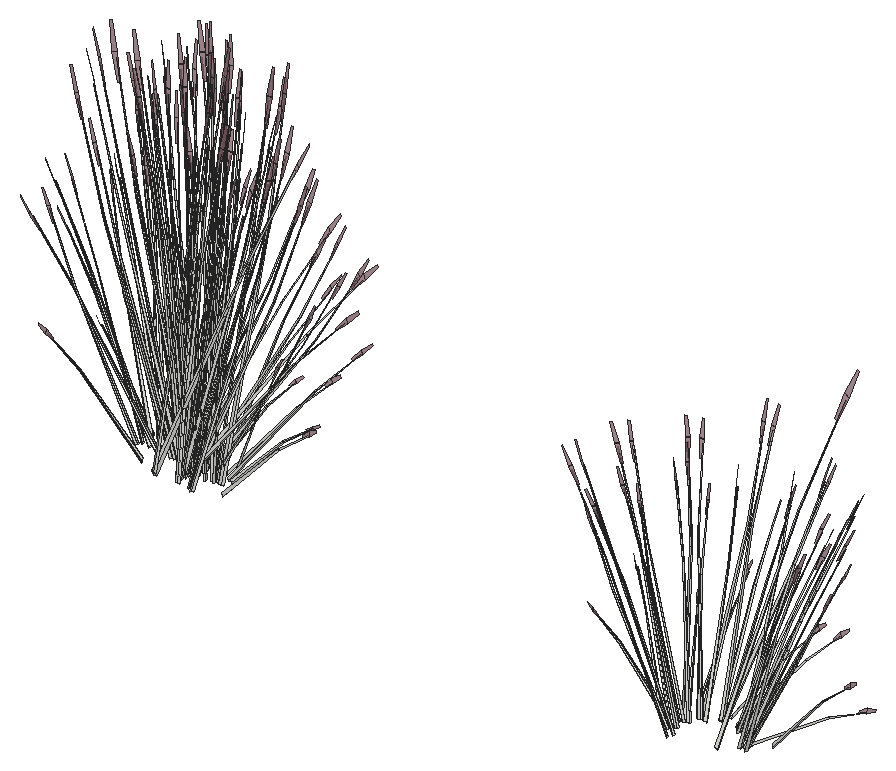
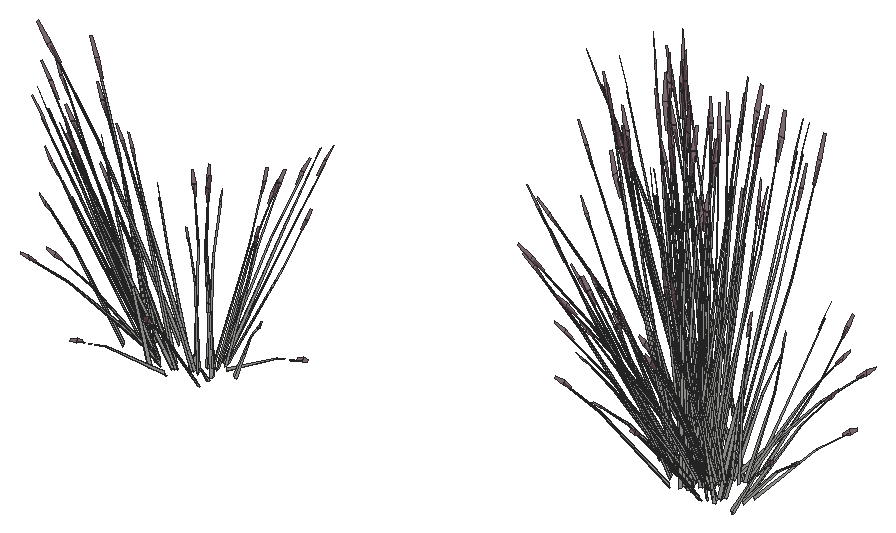
# SketchUp Ruby script. Lengths in millimetres.
U = 1.mm
M = Sketchup.active_model
def pt(a) = Geom::Point3d.new(a.map { |v| v * U })
def face(e, loops, mat)
  f = e.add_face(loops[0].map { |a| pt(a) })
  loops[1..].each { |l| e.add_face(l.map { |a| pt(a) }).erase! }
  f.material = f.back_material = mat if mat
  f
end
# faces: each face lists its corners as indices into pts; further lists are holes
def faces(e, pts, list, mat = nil) = list.each { |f| face(e, (f[0].is_a?(Array) ? f : [f]).map { |l| l.map { |i| pts[i] } }, mat) }
# xy, xz, yz: faces in a plane at the given z, y or x. An outline is a flat list of corners, or four numbers for a rectangle; further outlines are holes
def ring(l) = l.size == 4 ? [[l[0], l[1]], [l[2], l[1]], [l[2], l[3]], [l[0], l[3]]] : l.each_slice(2).to_a
def flat(e, list, mat, &to3) = list.each { |f| face(e, (f[0].is_a?(Array) ? f : [f]).map { |l| ring(l).map { |u, v| to3.(u, v) } }, mat) }
def xy(e, z, list, mat = nil) = flat(e, list, mat) { |x, y| [x, y, z] }
def xz(e, y, list, mat = nil) = flat(e, list, mat) { |x, z| [x, y, z] }
def yz(e, x, list, mat = nil) = flat(e, list, mat) { |y, z| [x, y, z] }
def lines(e, pts, list) = list.each { |a, b| e.add_line(pt(pts[a]), pt(pts[b])) }
# prism: a flat outline (further loops are holes) pulled along v
def prism(e, loops, v, mat = nil)
  f = face(e, loops, mat); d = Geom::Vector3d.new(v.map { |x| x * U })
  f.pushpull(f.normal.samedirection?(d) ? d.length : -d.length)
end
def box(e, o, s, mat = nil) = prism(e, [[o, [o[0] + s[0], o[1], o[2]], [o[0] + s[0], o[1] + s[1], o[2]], [o[0], o[1] + s[1], o[2]]]], [0, 0, s[2]], mat)
def at(x, y, z, deg = 0) = Geom::Transformation.translation(pt([x, y, z])) * Geom::Transformation.rotation(ORIGIN, Z_AXIS, deg.degrees)
def axes(o, x, y, z) = Geom::Transformation.new([*x, 0, *y, 0, *z, 0, *pt(o).to_a, 1])
def part(name) = M.definitions.add(name)
# library, detail: a bought-in or finely detailed component or shape, given as its bounding box
def library(name, o, s) = part(name).tap { |d| box(d.entities, o, s) }
def detail(e, o, s) = box(e.add_group.entities, o, s)
def put(e, d, t, mat = nil) = e.add_instance(d, t).tap { |i| i.material = mat if mat }
def group(e, t, mat = nil) = e.add_group.tap { |g| g.transformation = t; g.material = mat if mat }.entities
root = M.entities
M.materials.add("LightPink_Translucent").color = [144, 107, 117]
M.materials["LightPink_Translucent"].alpha = 0.8
c1 = part("blade")
p = [[54.7,5.3,558.8],[0,4.4,0],[2.3,11.5,0],[55.5,7.8,558.8],[58.2,7.8,558.8],[9.8,11.5,0],
  [62.9,5.7,838.2],[63,6,838.2],[63.4,6,838.2]]
faces(c1.entities,p,[[0,1,2,3],[4,5,2,3],[6,0,3,7],[7,3,4,8]])
c2 = part("seeds")
p = [[7.6,-2.7,35.1],[-0.2,-0.6,40.4],[-0.2,-0.8,0.9],[3.5,-1.8,-1.7],[7.5,-0.8,76.3],[3.7,0.2,78.9]]
faces(c2.entities,p,[[0,1,2,3],[1,0,4,5]],"LightPink_Translucent")
c3 = part("blade with seeds")
put(c3.entities,c1,at(0,0,0))
put(c3.entities,c2,axes([60.9,6.5,787.2],[1.5799,-0.05474,1.17369],[-0.12525,1.92788,0.29478],[-0.07173,-0.02425,1.56792]))
put(root,c3,axes([14135.3,12550.9,8467.4],[-0.35402,1.02926,0.17642],[-1.29548,-0.29127,0.35086],[0.22379,-0.00501,1.60407]))
put(root,c3,axes([14121.7,12572,8445],[-1.20625,0.41464,1.28929],[-0.38394,-1.1897,0.50096],[0.74071,0.01979,1.46642]))
put(root,c3,axes([16236.2,12606.2,8205.5],[0.69728,0.64842,0.35414],[-0.79619,0.61382,-0.4572],[-0.40453,-0.09339,0.87481]))
put(root,c3,axes([14204,12580,8471],[0.23642,-0.92427,0.1448],[1.15506,0.16044,-0.41347],[0.21021,0.09491,1.26744]))
put(root,c3,axes([14153.3,12635.7,8464.5],[1.54892,0.2182,0.45755],[-0.31522,1.23236,0.17955],[-0.22636,-0.119,1.58856]))
put(root,c3,axes([14361,12613,8442.4],[-0.06405,-0.15723,1.76342],[0.44421,-0.91974,-0.26939],[0.4481,-0.01323,0.30037]))
put(root,c3,axes([14025.1,12609,8442.4],[0.03108,0.16322,1.76342],[-0.62654,0.85237,-0.26939],[-0.44504,-0.04296,0.30037]))
put(root,c3,axes([16231.3,12595.7,8205.1],[-0.06562,1.05324,-0.1216],[-1.2424,-0.02879,-0.67495],[-0.4785,-0.07316,1.02557]))
put(root,c3,axes([14191.5,12586.1,8473.6],[-0.73619,-0.86927,0.44739],[1.11511,-0.61213,-0.21531],[0.23824,0.10756,1.43643]))
put(root,c3,axes([16467.5,12698.4,8205.1],[-0.6166,-0.93779,-0.1216],[1.09436,-0.46085,-0.67495],[0.46117,-0.12373,1.02557]))
put(root,c3,axes([14094.9,12687.1,8456],[-0.28787,-0.90242,-0.30978],[1.14332,-0.25625,0.30978],[-0.23049,-0.10406,1.38974]))
put(root,c3,axes([14132.2,12685.7,8467.4],[1.31687,-0.27488,0.17642],[0.32517,1.02297,0.35086],[-0.11745,-0.14905,1.60407]))
put(root,c3,axes([14201.1,12587.6,8472.2],[1.23732,-0.68758,-0.29095],[0.8228,0.97154,-0.50002],[0.30528,0.09867,1.59708]))
put(root,c3,axes([14326,12633.6,8519.5],[1.01846,0.28891,-0.35414],[-0.29705,0.84289,0.4572],[0.41005,-0.07729,0.87481]))
put(root,c3,axes([14086.7,12696.9,8455.8],[-1.14694,-0.51783,-0.49651],[0.68554,-0.92854,0],[-0.26122,-0.11794,1.57504]))
put(root,c3,axes([14280.3,12541.2,8455.8],[1.14694,0.51783,-0.49651],[-0.68554,0.92854,0],[0.26122,0.11794,1.57504]))
put(root,c3,axes([14021.9,12599.5,8519.5],[-1.01846,-0.28891,-0.35414],[0.29705,-0.84289,0.4572],[-0.41005,0.07729,0.87481]))
put(root,c3,axes([14225,12616.2,8460.5],[1.37109,0,0],[0,1.07219,0],[0,0,1.78407]))
put(root,c3,axes([14166,12650.5,8472.2],[-1.23732,0.68758,-0.29095],[-0.8228,-0.97154,-0.50002],[-0.30528,-0.09867,1.59708]))
put(root,c3,axes([14234.9,12552.3,8467.4],[-1.31687,0.27488,0.17642],[-0.32517,-1.02297,0.35086],[0.11745,0.14905,1.60407]))
put(root,c3,axes([14255.5,12607.1,8503],[-0.50831,0.02346,1.71376],[0.33721,-1.01661,0.13857],[0.72439,0.06288,0.73262]))
put(root,c3,axes([14272.2,12551,8456],[0.28787,0.90242,-0.30978],[-1.14332,0.25625,0.30978],[0.23049,0.10406,1.38974]))
put(root,c3,axes([16456.6,12691.2,8205.5],[-1.01846,-0.28891,0.35414],[0.29705,-0.84289,-0.4572],[0.41005,-0.07729,0.87481]))
put(root,c3,axes([14213.7,12602.3,8465],[-1.54892,-0.2182,0.49198],[0.31522,-1.23236,0.19306],[0.22636,0.119,1.70813]))
put(root,c3,axes([14182.4,12679.6,8460.5],[-0.39985,-0.89288,0],[1.1418,-0.31268,0],[0,0,1.54371]))
put(root,c3,axes([16185.8,12652.1,8197.4],[0.34623,-0.9443,0.48003],[1.13828,0.3229,0.3958],[-0.44763,0.05675,0.9933]))
put(root,c3,axes([14163,12658.1,8471],[-0.23642,0.92427,0.1448],[-1.15506,-0.16044,-0.41347],[-0.21021,-0.09491,1.26744]))
put(root,c3,axes([16183.6,12645.7,8197.4],[-0.4501,-0.70615,0.0643],[0.82077,-0.34564,0.50621],[-0.36181,0.0682,0.77189]))
put(root,c3,axes([14220.4,12676.4,8460],[1.2866,-0.3514,-0.19198],[0.45209,1.01223,0.00008],[0.14202,-0.03884,1.73897]))
put(root,c3,axes([14231.7,12687.2,8467.4],[0.35402,-1.02926,0.17642],[1.29548,0.29127,0.35086],[-0.22379,0.00501,1.60407]))
put(root,c3,axes([14224.2,12627.9,8460.8],[0.85545,0.66896,0],[-0.85545,0.66896,0],[0,0,1.69266]))
put(root,c3,axes([14100.7,12596,8489.4],[0.34834,-0.14982,1.77064],[0.12012,1.04605,0.13857],[-0.75452,0.1388,0.63284]))
put(root,c3,axes([14283.1,12620.5,8467.4],[-0.96285,-0.75439,0.17642],[0.97031,-0.7317,0.35086],[-0.10634,0.15406,1.60407]))
put(root,c3,axes([14237.8,12591.5,8456.8],[1.27479,0.1698,-0.62353],[-0.26901,1.04736,-0.16365],[0.38043,0.12691,1.37633]))
put(root,c3,axes([14380.9,12638,8474.7],[-0.75718,0.17097,1.1486],[0.35641,-0.70661,0.84392],[0.40168,0.04835,0.25299]))
put(root,c3,axes([14175.2,12689.9,8460.3],[-1.23546,-0.46496,0],[0.59459,-0.96613,0],[0,0,1.62707]))
put(root,c3,axes([14201.3,12658.4,8467.1],[-1.19666,-0.83357,-0.25192],[1.00694,-0.93603,0.5513],[-0.32224,0.09751,1.68216]))
put(root,c3,axes([14121.3,12699,8467.5],[1.14694,0.51783,0.49651],[-0.68554,0.92854,0],[-0.26122,-0.11794,1.57504]))
put(root,c3,axes([14223.9,12608,8473.6],[0.59459,-0.93321,0.44739],[1.23546,0.44912,-0.21531],[0,0.21512,1.43643]))
put(root,c3,axes([14218.1,12621.5,8462.7],[0,1.19774,-0.05637],[-1.53239,0,0],[0,0.03764,1.79368]))
put(root,c3,axes([14039.7,12610.5,8523.4],[-0.332,0.94205,-0.51099],[-1.13828,-0.3229,-0.3958],[-0.45829,0.08638,0.97773]))
put(root,c3,axes([14221,12600,8460.7],[0.73619,0.86927,-0.44739],[-1.11511,0.61213,0.21531],[0.23824,0.10756,1.43643]))
put(root,c3,axes([14347.4,12693.3,8504.3],[-0.23455,-0.87059,-0.03492],[1.10861,-0.20015,-0.15832],[0.23151,0.05519,0.52218]))
put(root,c3,axes([14104.5,12712.8,8464.8],[-0.7662,1.03778,0],[-1.28187,-0.57875,-0.51607],[-0.29196,-0.13181,1.63711]))
put(root,c3,axes([14303.2,12621.2,8467.5],[0,-1.03566,0.49651],[1.37109,0,0],[0,0.23588,1.57504]))
put(root,c3,axes([14215.9,12640.9,8473.6],[1.33077,-0.06393,0.44739],[0.12035,1.06125,-0.21531],[-0.23824,0.10756,1.43643]))
put(root,c3,axes([14237,12613.4,8471],[1.1418,-0.30203,0.1448],[0.39985,0.86246,-0.41347],[0,0.18981,1.26744]))
put(root,c3,axes([16480,12697.9,8197.4],[0.4501,0.70615,0.0643],[-0.82077,0.34564,0.50621],[0.36181,-0.0682,0.77189]))
put(root,c3,axes([16477.8,12691.5,8197.4],[-0.34623,0.9443,0.48003],[-1.13828,-0.3229,0.3958],[0.44763,-0.05675,0.9933]))
put(root,c3,axes([14185.9,12653.9,8460.7],[-1.33077,0.06393,-0.44739],[-0.12035,-1.06125,0.21531],[-0.23824,0.10756,1.43643]))
put(root,c3,axes([16207,12652.4,8205.5],[1.01846,0.28891,0.35414],[-0.29705,0.84289,-0.4572],[-0.41005,0.07729,0.87481]))
put(root,c3,axes([14344.8,12666.8,8470.3],[-0.29514,-0.25472,1.43002],[0.38401,-0.84262,-0.30754],[0.59714,0.11414,0.61141]))
put(root,c3,axes([14210.8,12690.3,8460.5],[1.23546,0.46496,0],[-0.59459,0.96613,0],[0,0,1.74954]))
put(root,c3,axes([14223.3,12716.4,8460.2],[-0.75665,-1.04141,-0.05142],[1.28187,-0.57875,0.51607],[-0.31588,0.09915,1.6363]))
put(root,c3,axes([14216.5,12652.5,8471],[0.90538,0.62224,0.1448],[-0.75521,0.70202,-0.41347],[-0.21021,0.09491,1.26744]))
put(root,c3,axes([14038.7,12622.8,8503],[0.42521,-0.21906,1.71376],[0.35798,1.01226,0.13857],[-0.66754,0.22878,0.73262]))
put(root,c3,axes([16529.8,12769.1,8196.8],[-0.11081,-0.09067,1.77383],[0.2424,-0.97188,-0.16761],[0.43649,-0.06209,0.31391]))
put(root,c3,axes([14276,12679.8,8531],[1.22504,0.02494,-0.71045],[-0.08228,1.05005,0.08574],[0.51899,0.11081,1.00501]))
put(root,c3,axes([16163.5,12669,8197],[-0.20012,0.13446,1.74944],[0.01702,0.98243,-0.27667],[-0.45871,0.12776,0.14031]))
put(root,c3,axes([16196.1,12645.2,8205.1],[0.6166,0.93779,-0.1216],[-1.09436,0.46085,-0.67495],[-0.46117,0.12373,1.02557]))
put(root,c3,axes([14241,12701.2,8467.5],[1.14694,-0.51783,0.49651],[0.68554,0.92854,0],[-0.26122,0.11794,1.57504]))
put(root,c3,axes([16432.3,12747.9,8205.1],[0.06562,-1.05324,-0.1216],[1.2424,0.02879,-0.67495],[0.4785,0.07316,1.02557]))
put(root,c3,axes([14199.5,12680.4,8462.7],[0.53281,1.18979,-0.06012],[-1.52239,0.41691,0],[0.01861,0.04155,1.72173]))
put(root,c3,axes([14214.5,12713.1,8456],[-1.14332,-0.25625,-0.30978],[0.28787,-0.90242,0.30978],[-0.23049,0.10406,1.38974]))
put(root,c3,axes([14005,12666.6,8470.3],[0.42589,0.08502,1.43002],[0.2745,0.86839,-0.30754],[-0.57851,0.16255,0.61141]))
put(root,c3,axes([14326.8,12625.7,8464.9],[1.53239,0,0],[0,1.1575,-0.51607],[0,0.26363,1.63711]))
put(root,c3,axes([16427.5,12737.4,8205.5],[-0.69728,-0.64842,0.35414],[0.79619,-0.61382,-0.4572],[0.40453,0.09339,0.87481]))
put(root,c3,axes([14311.3,12640.8,8460.4],[-1.53164,-0.00828,-0.04976],[0,-1.1575,0.49943],[-0.04813,0.2635,1.58352]))
put(root,c3,axes([14227.1,12615.2,8472.2],[1.38012,0.49416,-0.29095],[-0.66454,1.04299,-0.50002],[0.04337,0.25608,1.59708]))
put(root,c3,axes([13982.5,12712.8,8474.7],[0.51072,-0.46938,1.1486],[0.20153,0.74307,0.84392],[-0.36908,0.13305,0.25299]))
put(root,c3,axes([14294.7,12690.8,8519.5],[0.69728,0.64842,-0.35414],[-0.79619,0.61382,0.4572],[0.40453,0.09339,0.87481]))
put(root,c3,axes([14303.2,12645.1,8456],[-0.85545,0.64616,-0.30978],[-0.85545,-0.64616,0.30978],[0,0.20813,1.38974]))
put(root,c3,axes([14209.6,12646.6,8472.2],[0.1428,1.18174,-0.29095],[-1.48733,0.07145,-0.50002],[-0.26191,0.15741,1.59708]))
put(root,c3,axes([14223.3,12634.9,8460.7],[-0.59459,0.93321,-0.44739],[-1.23546,-0.44912,0.21531],[0,0.21512,1.43643]))
put(root,c3,axes([14031.4,12661.3,8519.5],[-1.06674,0.14801,-0.35414],[-0.28168,-0.84611,0.4572],[-0.30569,0.22726,0.87481]))
put(root,c3,axes([16459.8,12731.8,8197],[0.26289,-0.01751,1.74944],[0.72108,-0.8046,-0.27667],[0.46761,0.10621,0.14031]))
put(root,c3,axes([16192.8,12711.8,8197.4],[-0.30393,-0.95317,0.48003],[1.19224,-0.16542,0.3958],[-0.35138,0.22417,0.9933]))
put(root,c3,axes([16186.8,12707.2,8197.4],[-0.8413,-0.43556,0.0643],[0.48981,-0.62025,0.50621],[-0.26973,0.20053,0.77189]))
put(root,c3,axes([14186.8,12669.6,8456.8],[-0.82544,0.77843,-0.62353],[-1.0254,-0.70586,-0.16365],[-0.33076,0.19418,1.37633]))
put(root,c3,axes([14224.2,12702.9,8463.7],[1.53422,0.33662,0.30756],[-0.38383,1.20322,-0.36492],[-0.25393,0.15059,1.64885]))
put(root,c3,axes([14221.4,12723.5,8455.8],[-1.14694,0.51783,-0.49651],[-0.68554,-0.92854,0],[-0.26122,0.11794,1.57504]))
put(root,c3,axes([14318.1,12645.6,8455.8],[0,1.03566,-0.49651],[-1.37109,0,0],[0,0.23588,1.57504]))
put(root,c3,axes([14231.1,12648.6,8503],[-0.45521,-0.17844,1.71376],[0.94204,-0.74856,0.13857],[0.58713,0.33769,0.73262]))
put(root,c3,axes([14273.9,12700.2,8474.7],[-0.69001,-0.29779,1.1486],[0.89096,-0.30257,0.84392],[0.24031,0.2563,0.25299]))
put(root,c3,axes([16211.3,12703.8,8205.5],[1.06674,-0.14801,0.35414],[0.28168,0.84611,-0.4572],[-0.30569,0.22726,0.87481]))
put(root,c3,axes([16107,12694.2,8196.8],[0.1564,0.02778,1.77383],[0.48382,0.91506,-0.16761],[-0.32016,0.24017,0.31391]))
put(root,c3,axes([14078.2,12640.1,8503],[0.30609,-0.31822,1.71376],[0.77286,0.85893,0.13857],[-0.53009,0.39116,0.73262]))
put(root,c3,axes([14053.7,12663.8,8523.4],[0.31482,0.94565,-0.51099],[-1.19224,0.16542,-0.3958],[-0.34166,0.254,0.97773]))
put(root,c3,axes([16443.5,12752.3,8197.4],[-0.06171,0.78753,0.0643],[-0.9318,-0.02159,0.50621],[0.35694,0.08241,0.77189]))
put(root,c3,axes([14247.8,12719.4,8464.8],[0.7662,1.03778,0],[-1.28187,0.57875,-0.51607],[-0.29196,0.13181,1.63711]))
put(root,c3,axes([16445.7,12745.9,8197.4],[-0.90362,0.68241,0.48003],[-0.77932,-0.72471,0.3958],[0.42395,0.12588,0.9933]))
put(root,c3,axes([14278.8,12728.3,8442.4],[0.08928,-0.14952,1.76342],[1.12407,-0.44035,-0.26939],[0.34078,0.22791,0.30037]))
put(root,c3,axes([14231.2,12615.1,8476.7],[-0.03348,-0.97511,1.41272],[1.51511,0.25277,0.59816],[-0.35835,0.53357,1.3335]))
put(root,c3,axes([14241.1,12642,8457.7],[0.44936,0.94823,-0.69212],[-1.29441,0.3415,-0.18165],[0.04967,0.32109,1.52773]))
put(root,c3,axes([14016.6,12725.1,8442.4],[0.16438,0.10347,1.76342],[0.27873,0.95868,-0.26939],[-0.36432,0.20444,0.30037]))
put(root,c3,axes([14234.3,12710.6,8523.4],[1.20928,-0.24619,-0.51099],[0.21154,0.93233,-0.3958],[0.32481,0.26718,0.97773]))
put(root,c3,axes([16149.8,12764.8,8220.6],[1.08141,0.27645,-0.06488],[-0.33265,0.85086,-0.29416],[-0.17688,0.12919,0.97024]))
put(root,c3,axes([14276.7,12734.6,8472.3],[-0.78586,-0.03248,1.0506],[0.51898,-0.68985,0.58006],[0.31045,0.24509,0.8241]))
put(root,c3,axes([16372.7,12766,8205.5],[-0.18927,-0.83419,0.35414],[1.08199,-0.22027,-0.4572],[0.29062,0.23905,0.87481]))
put(root,c3,axes([16391.2,12644.1,8190.8],[-1.05895,-0.53811,1.38283],[1.11816,-0.83781,0.59665],[0.34166,0.5049,1.33663]))
put(root,c3,axes([16197.3,12701.8,8205.1],[1.1336,0.57106,-0.1216],[-0.65308,0.827,-0.67495],[-0.32027,0.28747,1.02557]))
put(root,c3,axes([14072.3,12660,8503],[0.22818,-0.35597,1.71376],[0.95725,0.73667,0.13857],[-0.43183,0.45914,0.73262]))
put(root,c3,axes([16370.2,12777,8205.1],[0.73026,-0.88648,-0.1216],[1.05755,0.51071,-0.67495],[0.36761,0.25045,1.02557]))
put(root,c3,axes([14211.5,12692.1,8470.3],[0.02163,-0.34331,1.43002],[1.03345,-0.38348,-0.30754],[0.31903,0.4109,0.61141]))
put(root,c3,axes([14079.1,12711,8519.5],[-0.82919,0.54528,-0.35414],[-0.78493,-0.62262,0.4572],[-0.11943,0.31634,0.87481]))
put(root,c3,axes([16247.9,12746.6,8205.5],[0.82919,-0.54528,0.35414],[0.78493,0.62262,-0.4572],[-0.11943,0.31634,0.87481]))
put(root,c3,axes([16345.9,12795.7,8196.8],[0.00363,-0.12539,1.77383],[1.0502,-0.55319,-0.16761],[0.36479,0.19745,0.31391]))
put(root,c3,axes([14092.5,12764.8,8474.7],[-0.03171,-0.6158,1.1486],[0.7925,0.43922,0.84392],[-0.15586,0.29352,0.25299]))
put(root,c3,axes([16228.8,12759.1,8197.4],[-1.00708,-0.04826,0.0643],[0.02761,-0.72867,0.50621],[-0.10538,0.27912,0.77189]))
put(root,c3,axes([16237,12760.8,8197.4],[-0.87265,-0.70663,0.48003],[0.92674,-0.60943,0.3958],[-0.16097,0.33153,0.9933]))
put(root,c3,axes([14145.5,12727.5,8442.4],[0.19833,-0.05635,1.76342],[1.19302,0.31018,-0.26939],[0.03489,0.3496,0.30037]))
put(root,c3,axes([16307,12769.4,8205.5],[0.36946,-0.79643,0.35414],[1.07787,0.23229,-0.4572],[0.09883,0.32066,0.87481]))
put(root,c3,axes([14100,12704.5,8531.6],[0.87728,0.69587,-0.5672],[-0.92674,0.60943,-0.43934],[-0.13348,0.35356,1.08528]))
put(root,c3,axes([14075.8,12731,8476.2],[1.11329,-0.1834,0.06507],[0.25594,0.73887,-0.86304],[-0.07058,0.37403,0.7736]))
put(root,c3,axes([14166.1,12721.6,8523.4],[1.20468,0.25962,-0.51099],[-0.41292,0.89013,-0.3958],[0.11046,0.35838,0.97773]))
put(root,c3,axes([14183.5,12674.9,8503],[-0.28013,-0.33252,1.71376],[1.29445,-0.27994,0.13857],[0.29256,0.52202,0.73262]))
put(root,c3,axes([16377.1,12785.2,8197.4],[-0.55698,0.6579,0.0643],[-0.79316,-0.38303,0.50621],[0.25643,0.21093,0.77189]))
put(root,c3,axes([16343.8,12841.5,8220.6],[0.84686,-0.59414,-0.06488],[0.77596,0.65071,-0.29416],[0.05463,0.18438,0.97024]))
put(root,c3,axes([16383,12780.5,8197.4],[-1.21888,0.23767,0.48003],[-0.21154,-0.93233,0.3958],[0.28666,0.27478,0.9933]))
put(root,c3,axes([14152.1,12735.5,8519.5],[-0.36946,0.79643,-0.35414],[-1.07787,-0.23229,0.4572],[0.09883,0.32066,0.87481]))
put(root,c3,axes([14093.1,12696.4,8540.1],[-0.03189,0.95798,-0.7886],[-1.34277,-0.06434,0.09517],[-0.14171,0.40585,1.11556]))
put(root,c3,axes([14125.4,12679.1,8503],[-0.02999,-0.3975,1.71376],[1.30002,0.26369,0.13857],[-0.08041,0.56647,0.73262]))
put(root,c3,axes([16298.5,12787.7,8197.4],[-0.90301,0.35198,0.0643],[-0.44199,-0.64184,0.50621],[0.08721,0.28293,0.77189]))
put(root,c3,axes([16164.3,12762.1,8197],[-0.03046,0.20495,1.74944],[0.86449,0.71297,-0.27667],[-0.22632,0.33716,0.14031]))
put(root,c3,axes([16234.5,12750.4,8214.3],[1.34686,0.05131,-0.13498],[-0.03681,0.97156,-0.74919],[-0.09356,0.37418,1.13838]))
put(root,c3,axes([16297.8,12777.9,8205.1],[1.19922,-0.48218,-0.1216],[0.58932,0.85579,-0.67495],[0.15822,0.36063,1.02557]))
put(root,c3,axes([16306.6,12786,8205.8],[-1.20755,-0.27075,0.53283],[0.41292,-0.89013,0.43934],[0.07257,0.35005,1.10256]))
put(root,c3,axes([14155,12717.3,8531],[0.5849,0.8421,-0.71045],[-1.20401,0.4693,0.08574],[0.13677,0.40688,1.00501]))
put(root,c3,axes([14069,12751,8470.3],[0.38672,-0.16338,1.43002],[0.95481,0.49262,-0.30754],[-0.28419,0.42626,0.61141]))
put(root,c3,axes([14081.7,12730.7,8489.9],[0.02693,-0.53464,1.54345],[1.21102,0.2824,0.21329],[-0.10493,0.5698,0.72882]))
put(root,c3,axes([16161.8,12815.5,8196.8],[0.13903,-0.06253,1.77383],[1.14912,0.41591,-0.16761],[-0.027,0.34629,0.31391]))
put(root,c3,axes([16290.6,12826.5,8197],[0.15534,0.16677,1.74944],[1.25362,0.06552,-0.27667],[0.12606,0.3678,0.14031]))
